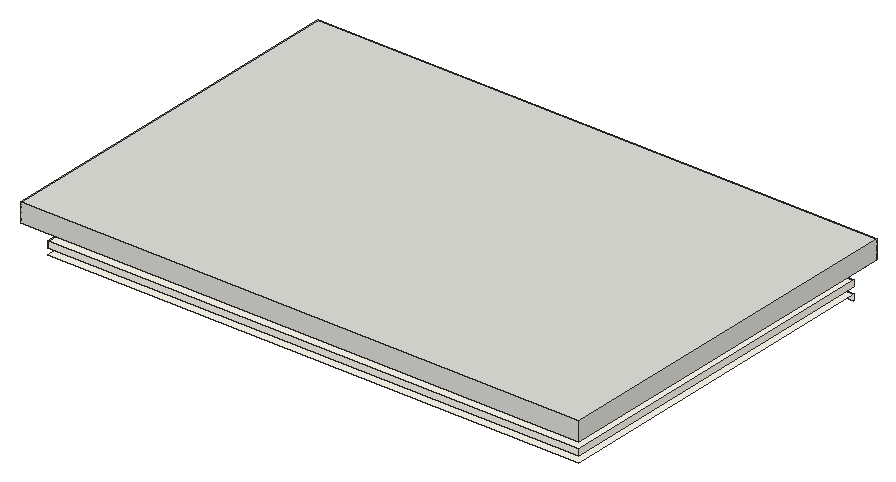
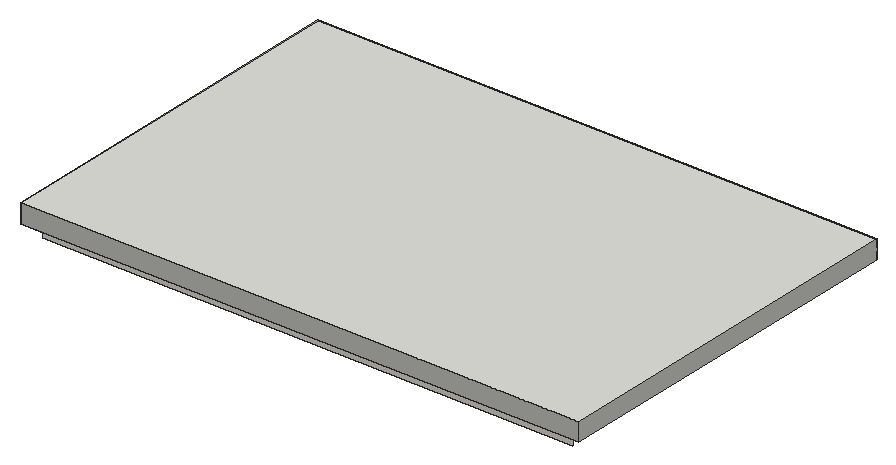
# SketchUp Ruby script. Lengths in inches.
U = 1.inch
M = Sketchup.active_model
def pt(a) = Geom::Point3d.new(a.map { |v| v * U })
def face(e, loops, mat)
  f = e.add_face(loops[0].map { |a| pt(a) })
  loops[1..].each { |l| e.add_face(l.map { |a| pt(a) }).erase! }
  f.material = f.back_material = mat if mat
  f
end
# faces: each face lists its corners as indices into pts; further lists are holes
def faces(e, pts, list, mat = nil) = list.each { |f| face(e, (f[0].is_a?(Array) ? f : [f]).map { |l| l.map { |i| pts[i] } }, mat) }
# xy, xz, yz: faces in a plane at the given z, y or x. An outline is a flat list of corners, or four numbers for a rectangle; further outlines are holes
def ring(l) = l.size == 4 ? [[l[0], l[1]], [l[2], l[1]], [l[2], l[3]], [l[0], l[3]]] : l.each_slice(2).to_a
def flat(e, list, mat, &to3) = list.each { |f| face(e, (f[0].is_a?(Array) ? f : [f]).map { |l| ring(l).map { |u, v| to3.(u, v) } }, mat) }
def xy(e, z, list, mat = nil) = flat(e, list, mat) { |x, y| [x, y, z] }
def xz(e, y, list, mat = nil) = flat(e, list, mat) { |x, z| [x, y, z] }
def yz(e, x, list, mat = nil) = flat(e, list, mat) { |y, z| [x, y, z] }
def lines(e, pts, list) = list.each { |a, b| e.add_line(pt(pts[a]), pt(pts[b])) }
# prism: a flat outline (further loops are holes) pulled along v
def prism(e, loops, v, mat = nil)
  f = face(e, loops, mat); d = Geom::Vector3d.new(v.map { |x| x * U })
  f.pushpull(f.normal.samedirection?(d) ? d.length : -d.length)
end
def box(e, o, s, mat = nil) = prism(e, [[o, [o[0] + s[0], o[1], o[2]], [o[0] + s[0], o[1] + s[1], o[2]], [o[0], o[1] + s[1], o[2]]]], [0, 0, s[2]], mat)
def at(x, y, z, deg = 0) = Geom::Transformation.translation(pt([x, y, z])) * Geom::Transformation.rotation(ORIGIN, Z_AXIS, deg.degrees)
def axes(o, x, y, z) = Geom::Transformation.new([*x, 0, *y, 0, *z, 0, *pt(o).to_a, 1])
def part(name) = M.definitions.add(name)
# library, detail: a bought-in or finely detailed component or shape, given as its bounding box
def library(name, o, s) = part(name).tap { |d| box(d.entities, o, s) }
def detail(e, o, s) = box(e.add_group.entities, o, s)
def put(e, d, t, mat = nil) = e.add_instance(d, t).tap { |i| i.material = mat if mat }
def group(e, t, mat = nil) = e.add_group.tap { |g| g.transformation = t; g.material = mat if mat }.entities
root = M.entities
M.materials.add("[0052_FloralWhite]").color = [255, 250, 240]
M.materials.add("[Color D02]").color = [214, 192, 128]
M.materials.add("[Color E02]").color = [255, 255, 153]
M.materials.add("[Metal Aluminum Anodized]").color = [202, 209, 219]
xy(root,118.125,[[[49.94,94.53,49.875,94.55,49.81,94.5625,49.74,94.58,49.67,94.61,49.61,94.64,49.55,94.68,49.49,94.71,49.4375,94.76,49.39,94.8,49.34,94.85,49.29,94.91,49.25,94.96,49.21,95.02,49.18,95.08,49.15,95.15,49.13,95.21,49.09,95.35,49.08,95.42,49.08,95.63,49.09,95.7,49.11,95.76,49.15,95.9,49.21,96.02,49.29,96.14,49.33,96.19,49.43,96.29,49.61,96.41,49.67,96.4375,49.73,96.46,49.8,96.49,49.87,96.5,49.9375,96.51,50.01,96.52,50.22,96.52,50.28,96.5,50.35,96.49,50.42,96.47,50.48,96.44,50.55,96.41,50.61,96.375,50.66,96.34,50.72,96.29,50.77,96.25,50.82,96.2,50.87,96.14,50.91,96.09,50.94,96.03,50.98,95.97,51.01,95.9,51.03,95.84,51.05,95.77,51.0625,95.7,51.07,95.63,51.08,95.5625,51.08,95.49,51.07,95.42,51.0625,95.35,51.05,95.29,51.01,95.15,50.95,95.03,50.87,94.91,50.82,94.86,50.78,94.81,50.72,94.76,50.67,94.72,50.55,94.64,50.49,94.61,50.42,94.59,50.36,94.5625,50.29,94.55,50.15,94.53],[50.02,94.7,50.14,94.7,50.2,94.71,50.25,94.72,50.31,94.73,50.36,94.75,50.42,94.77,50.52,94.83,50.56,94.86,50.61,94.9,50.65,94.93,50.69,94.98,50.73,95.02,50.76,95.07,50.79,95.11,50.82,95.17,50.86,95.27,50.88,95.33,50.89,95.38,50.9,95.44,50.9,95.61,50.88,95.73,50.86,95.78,50.84,95.84,50.82,95.89,50.79,95.9375,50.76,95.99,50.73,96.03,50.69,96.08,50.61,96.16,50.5625,96.19,50.51,96.22,50.41,96.28,50.36,96.3,50.3,96.32,50.25,96.33,50.13,96.35,50.02,96.35,49.96,96.34,49.91,96.33,49.85,96.32,49.8,96.3,49.74,96.28,49.59,96.19,49.55,96.15,49.5,96.12,49.47,96.07,49.43,96.03,49.39,95.98,49.36,95.94,49.34,95.88,49.3125,95.83,49.29,95.78,49.28,95.72,49.27,95.67,49.26,95.61,49.26,95.4375,49.27,95.38,49.28,95.32,49.3,95.27,49.32,95.21,49.34,95.16,49.37,95.11,49.4,95.0625,49.43,95.02,49.47,94.97,49.55,94.89,49.6,94.86,49.64,94.83,49.69,94.8,49.75,94.77,49.85,94.73,49.97,94.71]]],"[Metal Aluminum Anodized]")
xy(root,118.1875,[[50.02,94.7,49.97,94.71,49.85,94.73,49.75,94.77,49.69,94.8,49.64,94.83,49.6,94.86,49.55,94.89,49.47,94.97,49.43,95.02,49.4,95.0625,49.37,95.11,49.34,95.16,49.32,95.21,49.3,95.27,49.28,95.32,49.27,95.38,49.26,95.4375,49.26,95.61,49.27,95.67,49.28,95.72,49.29,95.78,49.3125,95.83,49.34,95.88,49.36,95.94,49.39,95.98,49.43,96.03,49.47,96.07,49.5,96.12,49.55,96.15,49.59,96.19,49.74,96.28,49.8,96.3,49.85,96.32,49.91,96.33,49.96,96.34,50.02,96.35,50.13,96.35,50.25,96.33,50.3,96.32,50.36,96.3,50.41,96.28,50.51,96.22,50.5625,96.19,50.61,96.16,50.69,96.08,50.73,96.03,50.76,95.99,50.79,95.9375,50.82,95.89,50.84,95.84,50.86,95.78,50.88,95.73,50.9,95.61,50.9,95.44,50.89,95.38,50.88,95.33,50.86,95.27,50.82,95.17,50.79,95.11,50.76,95.07,50.73,95.02,50.69,94.98,50.65,94.93,50.61,94.9,50.56,94.86,50.52,94.83,50.42,94.77,50.36,94.75,50.31,94.73,50.25,94.72,50.2,94.71,50.14,94.7]],"[Color D02]")
xy(root,118.3,[[[24.3,77.95,24.23,77.96,24.16,77.96,24.09,77.98,24.02,77.99,23.96,78.01,23.89,78.04,23.83,78.07,23.77,78.11,23.71,78.14,23.66,78.1875,23.61,78.23,23.56,78.28,23.51,78.34,23.47,78.39,23.43,78.45,23.4,78.52,23.37,78.58,23.35,78.64,23.33,78.71,23.3,78.92,23.3,78.99,23.33,79.2,23.35,79.26,23.37,79.33,23.43,79.45,23.51,79.57,23.66,79.72,23.71,79.76,23.83,79.84,23.89,79.87,23.96,79.89,24.02,79.92,24.23,79.95,24.37,79.95,24.4375,79.94,24.51,79.93,24.58,79.92,24.64,79.89,24.71,79.87,24.77,79.84,24.89,79.76,24.94,79.72,25.09,79.57,25.17,79.45,25.23,79.33,25.25,79.26,25.27,79.2,25.3,78.99,25.3,78.92,25.27,78.71,25.25,78.64,25.23,78.58,25.2,78.52,25.17,78.45,25.13,78.39,25.09,78.34,25.04,78.28,24.99,78.23,24.94,78.1875,24.89,78.14,24.83,78.11,24.77,78.07,24.71,78.04,24.64,78.01,24.58,77.99,24.51,77.98,24.4375,77.96,24.37,77.96],[24.23,78.02,24.37,78.02,24.49,78.04,24.56,78.06,24.68,78.1,24.74,78.13,24.79,78.16,24.85,78.2,24.95,78.28,24.99,78.33,25.04,78.38,25.07,78.43,25.11,78.49,25.14,78.54,25.16,78.6,25.1875,78.67,25.21,78.73,25.22,78.79,25.23,78.86,25.23,79.05,25.22,79.12,25.21,79.18,25.1875,79.24,25.16,79.3,25.14,79.36,25.11,79.42,25.07,79.48,25.04,79.53,24.99,79.58,24.95,79.625,24.9,79.67,24.85,79.71,24.79,79.74,24.74,79.78,24.68,79.81,24.56,79.85,24.49,79.87,24.43,79.88,24.37,79.88,24.3,79.89,24.23,79.88,24.17,79.88,24.11,79.87,24.04,79.85,23.92,79.81,23.86,79.78,23.81,79.74,23.75,79.71,23.7,79.67,23.65,79.625,23.61,79.58,23.56,79.53,23.53,79.48,23.49,79.42,23.46,79.36,23.44,79.3,23.41,79.24,23.39,79.18,23.38,79.12,23.37,79.05,23.37,78.86,23.38,78.79,23.39,78.73,23.41,78.67,23.44,78.6,23.46,78.54,23.49,78.49,23.53,78.43,23.56,78.38,23.61,78.33,23.65,78.28,23.75,78.2,23.81,78.16,23.86,78.13,23.92,78.1,24.04,78.06,24.11,78.04]]],"[Metal Aluminum Anodized]")
xy(root,118.375,[[24.23,78.02,24.11,78.04,24.04,78.06,23.92,78.1,23.86,78.13,23.81,78.16,23.75,78.2,23.65,78.28,23.61,78.33,23.56,78.38,23.53,78.43,23.49,78.49,23.46,78.54,23.44,78.6,23.41,78.67,23.39,78.73,23.38,78.79,23.37,78.86,23.37,79.05,23.38,79.12,23.39,79.18,23.41,79.24,23.44,79.3,23.46,79.36,23.49,79.42,23.53,79.48,23.56,79.53,23.61,79.58,23.65,79.625,23.7,79.67,23.75,79.71,23.81,79.74,23.86,79.78,23.92,79.81,24.04,79.85,24.11,79.87,24.17,79.88,24.23,79.88,24.3,79.89,24.37,79.88,24.43,79.88,24.49,79.87,24.56,79.85,24.68,79.81,24.74,79.78,24.79,79.74,24.85,79.71,24.9,79.67,24.95,79.625,24.99,79.58,25.04,79.53,25.07,79.48,25.11,79.42,25.14,79.36,25.16,79.3,25.1875,79.24,25.21,79.18,25.22,79.12,25.23,79.05,25.23,78.86,25.22,78.79,25.21,78.73,25.1875,78.67,25.16,78.6,25.14,78.54,25.11,78.49,25.07,78.43,25.04,78.38,24.99,78.33,24.95,78.28,24.85,78.2,24.79,78.16,24.74,78.13,24.68,78.1,24.56,78.06,24.49,78.04,24.37,78.02]],"[Color E02]")
xy(root,120,[[[9,0,180,111],[39.6,30.6,149.4,80.4]]],"[0052_FloralWhite]")
xz(root,78.02,[[24.23,118.3,24.3,118.375],[24.3,118.3,24.37,118.375]],"[0052_FloralWhite]")
xz(root,79.88,[[24.17,118.3,24.23,118.375],[24.37,118.3,24.43,118.375]],"[0052_FloralWhite]")
xz(root,79.95,[[24.23,118,24.3,118.3],[24.3,118,24.37,118.3]],"[Metal Aluminum Anodized]")
xz(root,94.7,[[50.02,118.125,50.08,118.1875],[50.08,118.125,50.14,118.1875]],"[Metal Aluminum Anodized]")
xz(root,96.35,[[50.02,118.125,50.08,118.1875],[50.08,118.125,50.13,118.1875]],"[Metal Aluminum Anodized]")
xz(root,111,[[9,118,180,120]],"[0052_FloralWhite]")
yz(root,23.37,[[78.86,118.3,78.92,118.375],[78.92,118.3,78.99,118.375],[78.99,118.3,79.05,118.375]],"[0052_FloralWhite]")
yz(root,25.23,[[78.86,118.3,78.92,118.375],[78.92,118.3,78.99,118.375],[78.99,118.3,79.05,118.375]],"[0052_FloralWhite]")
yz(root,49.26,[[95.4375,118.125,95.49,118.1875],[95.49,118.125,95.55,118.1875],[95.55,118.125,95.61,118.1875]],"[Metal Aluminum Anodized]")
yz(root,50.9,[[95.44,118.125,95.5,118.1875],[95.5,118.125,95.56,118.1875],[95.56,118.125,95.61,118.1875]],"[Metal Aluminum Anodized]")
p = [[23.66,79.72,118],[23.71,79.76,118],[23.71,79.76,118.3],[23.66,79.72,118.3],[24.89,79.76,118],[24.94,79.72,118],
  [24.94,79.72,118.3],[24.89,79.76,118.3],[23.77,79.8,118],[23.77,79.8,118.3],[23.83,79.84,118],[23.83,79.84,118.3],
  [23.89,79.87,118],[23.89,79.87,118.3],[24.71,79.87,118],[24.77,79.84,118],[24.77,79.84,118.3],[24.71,79.87,118.3],
  [24.83,79.8,118],[24.83,79.8,118.3],[23.96,79.89,118],[23.96,79.89,118.3],[24.02,79.92,118],[24.02,79.92,118.3],
  [24.09,79.93,118],[24.09,79.93,118.3],[24.16,79.94,118],[24.16,79.94,118.3],[24.23,79.95,118],[24.23,79.95,118.3],
  [24.37,79.95,118],[24.4375,79.94,118],[24.4375,79.94,118.3],[24.37,79.95,118.3],[24.51,79.93,118],[24.51,79.93,118.3],
  [24.58,79.92,118],[24.58,79.92,118.3],[24.64,79.89,118],[24.64,79.89,118.3],[49.8,94.75,118.1875],[49.8,94.75,118.125],
  [49.75,94.77,118.125],[49.75,94.77,118.1875],[49.85,94.73,118.1875],[49.85,94.73,118.125],[49.97,94.71,118.1875],[49.97,94.71,118.125],
  [49.91,94.72,118.125],[49.91,94.72,118.1875],[50.02,94.7,118.1875],[50.02,94.7,118.125],[50.2,94.71,118.1875],[50.2,94.71,118.125],
  [50.14,94.7,118.125],[50.14,94.7,118.1875],[50.25,94.72,118.1875],[50.25,94.72,118.125],[50.36,94.75,118.1875],[50.36,94.75,118.125],
  [50.31,94.73,118.125],[50.31,94.73,118.1875],[49.69,94.8,118.1875],[49.69,94.8,118.125],[49.64,94.83,118.125],[49.64,94.83,118.1875],
  [49.6,94.86,118.125],[49.6,94.86,118.1875],[50.47,94.8,118.1875],[50.47,94.8,118.125],[50.42,94.77,118.125],[50.42,94.77,118.1875],
  [50.56,94.86,118.1875],[50.56,94.86,118.125],[50.52,94.83,118.125],[50.52,94.83,118.1875],[49.55,94.89,118.1875],[49.55,94.89,118.125],
  [49.51,94.93,118.125],[49.51,94.93,118.1875],[49.47,94.97,118.125],[49.47,94.97,118.1875],[50.65,94.93,118.1875],[50.65,94.93,118.125],
  [50.61,94.9,118.125],[50.61,94.9,118.1875],[50.69,94.98,118.1875],[50.69,94.98,118.125],[49.43,95.02,118.125],[49.43,95.02,118.1875],
  [49.4,95.0625,118.125],[49.4,95.0625,118.1875],[50.76,95.07,118.1875],[50.76,95.07,118.125],[50.73,95.02,118.125],[50.73,95.02,118.1875],
  [49.37,95.11,118.1875],[49.37,95.11,118.125],[49.34,95.16,118.125],[49.34,95.16,118.1875],[50.82,95.17,118.1875],[50.82,95.17,118.125],
  [50.79,95.11,118.125],[50.79,95.11,118.1875],[49.32,95.21,118.125],[49.32,95.21,118.1875],[49.3,95.27,118.125],[49.3,95.27,118.1875],
  [50.86,95.27,118.1875],[50.86,95.27,118.125],[50.84,95.22,118.125],[50.84,95.22,118.1875],[49.28,95.32,118.125],[49.28,95.32,118.1875],
  [49.27,95.38,118.125],[49.27,95.38,118.1875],[50.89,95.38,118.1875],[50.89,95.38,118.125],[50.88,95.33,118.125],[50.88,95.33,118.1875],
  [49.26,95.4375,118.125],[49.26,95.4375,118.1875],[50.9,95.44,118.1875],[50.9,95.44,118.125],[49.26,95.61,118.1875],[49.26,95.61,118.125],
  [49.27,95.67,118.125],[49.27,95.67,118.1875],[50.89,95.67,118.1875],[50.89,95.67,118.125],[50.9,95.61,118.125],[50.9,95.61,118.1875],
  [49.28,95.72,118.125],[49.28,95.72,118.1875],[49.29,95.78,118.125],[49.29,95.78,118.1875],[50.86,95.78,118.1875],[50.86,95.78,118.125],
  [50.88,95.73,118.125],[50.88,95.73,118.1875],[49.3125,95.83,118.125],[49.3125,95.83,118.1875],[49.34,95.88,118.125],[49.34,95.88,118.1875],
  [50.82,95.89,118.1875],[50.82,95.89,118.125],[50.84,95.84,118.125],[50.84,95.84,118.1875],[49.36,95.94,118.125],[49.36,95.94,118.1875],
  [49.39,95.98,118.125],[49.39,95.98,118.1875],[50.76,95.99,118.1875],[50.76,95.99,118.125],[50.79,95.9375,118.125],[50.79,95.9375,118.1875],
  [49.43,96.03,118.125],[49.43,96.03,118.1875],[49.47,96.07,118.125],[49.47,96.07,118.1875],[50.69,96.08,118.1875],[50.69,96.08,118.125],
  [50.73,96.03,118.125],[50.73,96.03,118.1875],[49.5,96.12,118.125],[49.5,96.12,118.1875],[49.55,96.15,118.125],[49.55,96.15,118.1875],
  [50.61,96.16,118.1875],[50.61,96.16,118.125],[50.65,96.12,118.125],[50.65,96.12,118.1875],[49.59,96.19,118.125],[49.59,96.19,118.1875],
  [49.64,96.22,118.125],[49.64,96.22,118.1875],[49.69,96.25,118.125],[49.69,96.25,118.1875],[50.46,96.25,118.1875],[50.46,96.25,118.125],
  [50.51,96.22,118.125],[50.51,96.22,118.1875],[50.5625,96.19,118.125],[50.5625,96.19,118.1875],[49.74,96.28,118.125],[49.74,96.28,118.1875],
  [49.8,96.3,118.125],[49.8,96.3,118.1875],[49.85,96.32,118.125],[49.85,96.32,118.1875],[49.91,96.33,118.125],[49.91,96.33,118.1875],
  [49.96,96.34,118.125],[49.96,96.34,118.1875],[50.02,96.35,118.125],[50.02,96.35,118.1875],[50.13,96.35,118.1875],[50.13,96.35,118.125],
  [50.19,96.34,118.125],[50.19,96.34,118.1875],[50.25,96.33,118.125],[50.25,96.33,118.1875],[50.3,96.32,118.125],[50.3,96.32,118.1875],
  [50.36,96.3,118.125],[50.36,96.3,118.1875],[50.41,96.28,118.125],[50.41,96.28,118.1875],[24.11,78.04,118.375],[24.11,78.04,118.3],
  [24.04,78.06,118.3],[24.04,78.06,118.375],[24.17,78.03,118.375],[24.17,78.03,118.3],[24.23,78.02,118.375],[24.23,78.02,118.3],
  [24.49,78.04,118.375],[24.49,78.04,118.3],[24.43,78.03,118.3],[24.43,78.03,118.375],[24.37,78.02,118.3],[24.37,78.02,118.375],
  [24.56,78.06,118.375],[24.56,78.06,118.3],[23.86,78.13,118.375],[23.86,78.13,118.3],[23.81,78.16,118.3],[23.81,78.16,118.375],
  [23.98,78.08,118.375],[23.98,78.08,118.3],[23.92,78.1,118.3],[23.92,78.1,118.375],[24.68,78.1,118.375],[24.68,78.1,118.3],
  [24.62,78.08,118.3],[24.62,78.08,118.375],[24.79,78.16,118.375],[24.79,78.16,118.3],[24.74,78.13,118.3],[24.74,78.13,118.375],
  [23.75,78.2,118.375],[23.75,78.2,118.3],[23.7,78.24,118.3],[23.7,78.24,118.375],[23.65,78.28,118.3],[23.65,78.28,118.375],
  [24.9,78.24,118.375],[24.9,78.24,118.3],[24.85,78.2,118.3],[24.85,78.2,118.375],[24.95,78.28,118.375],[24.95,78.28,118.3],
  [23.61,78.33,118.3],[23.61,78.33,118.375],[23.56,78.38,118.3],[23.56,78.38,118.375],[24.99,78.33,118.375],[24.99,78.33,118.3],
  [25.04,78.38,118.375],[25.04,78.38,118.3],[23.53,78.43,118.3],[23.53,78.43,118.375],[23.49,78.49,118.3],[23.49,78.49,118.375],
  [25.07,78.43,118.375],[25.07,78.43,118.3],[25.11,78.49,118.375],[25.11,78.49,118.3],[23.46,78.54,118.375],[23.46,78.54,118.3],
  [23.44,78.6,118.3],[23.44,78.6,118.375],[25.16,78.6,118.375],[25.16,78.6,118.3],[25.14,78.54,118.3],[25.14,78.54,118.375],
  [23.41,78.67,118.3],[23.41,78.67,118.375],[25.1875,78.67,118.375],[25.1875,78.67,118.3],[23.39,78.73,118.3],[23.39,78.73,118.375],
  [23.38,78.79,118.3],[23.38,78.79,118.375],[25.21,78.73,118.375],[25.21,78.73,118.3],[25.22,78.79,118.375],[25.22,78.79,118.3],
  [23.37,78.86,118.3],[23.37,78.86,118.375],[25.23,78.86,118.375],[25.23,78.86,118.3],[23.37,79.05,118.375],[23.37,79.05,118.3],
  [23.38,79.12,118.3],[23.38,79.12,118.375],[23.39,79.18,118.3],[23.39,79.18,118.375],[25.21,79.18,118.375],[25.21,79.18,118.3],
  [25.22,79.12,118.3],[25.22,79.12,118.375],[25.23,79.05,118.3],[25.23,79.05,118.375],[23.41,79.24,118.3],[23.41,79.24,118.375],
  [23.44,79.3,118.3],[23.44,79.3,118.375],[25.1875,79.24,118.375],[25.1875,79.24,118.3],[25.16,79.3,118.375],[25.16,79.3,118.3],
  [23.46,79.36,118.3],[23.46,79.36,118.375],[25.14,79.36,118.375],[25.14,79.36,118.3],[23.49,79.42,118.3],[23.49,79.42,118.375],
  [23.53,79.48,118.3],[23.53,79.48,118.375],[25.07,79.48,118.375],[25.07,79.48,118.3],[25.11,79.42,118.3],[25.11,79.42,118.375],
  [23.56,79.53,118.3],[23.56,79.53,118.375],[23.61,79.58,118.3],[23.61,79.58,118.375],[24.99,79.58,118.375],[24.99,79.58,118.3],
  [25.04,79.53,118.3],[25.04,79.53,118.375],[23.65,79.625,118.3],[23.65,79.625,118.375],[23.7,79.67,118.3],[23.7,79.67,118.375],
  [24.9,79.67,118.375],[24.9,79.67,118.3],[24.95,79.625,118.3],[24.95,79.625,118.375],[23.75,79.71,118.3],[23.75,79.71,118.375],
  [23.81,79.74,118.3],[23.81,79.74,118.375],[23.86,79.78,118.3],[23.86,79.78,118.375],[24.74,79.78,118.375],[24.74,79.78,118.3],
  [24.79,79.74,118.3],[24.79,79.74,118.375],[24.85,79.71,118.3],[24.85,79.71,118.375],[23.92,79.81,118.3],[23.92,79.81,118.375],
  [23.98,79.83,118.3],[23.98,79.83,118.375],[24.04,79.85,118.3],[24.04,79.85,118.375],[24.56,79.85,118.375],[24.56,79.85,118.3],
  [24.62,79.83,118.3],[24.62,79.83,118.375],[24.68,79.81,118.3],[24.68,79.81,118.375],[24.11,79.87,118.3],[24.11,79.87,118.375],
  [24.17,79.88,118.3],[24.17,79.88,118.375],[24.23,79.88,118.375],[24.23,79.88,118.3],[24.3,79.89,118.3],[24.3,79.89,118.375],
  [24.37,79.88,118.3],[24.37,79.88,118.375],[24.43,79.88,118.375],[24.43,79.88,118.3],[24.49,79.87,118.3],[24.49,79.87,118.375]]
faces(root,p,[[0,1,2,3],[4,5,6,7],[1,8,9,2],[8,10,11,9],[10,12,13,11],[14,15,16,17],[15,18,19,16],[18,4,7,19],
  [12,20,21,13],[20,22,23,21],[22,24,25,23],[24,26,27,25],[26,28,29,27],[30,31,32,33],[31,34,35,32],[34,36,37,35],
  [36,38,39,37],[38,14,17,39],[40,41,42,43],[44,45,41,40],[46,47,48,49],[49,48,45,44],[50,51,47,46],[52,53,54,55],
  [56,57,53,52],[58,59,60,61],[61,60,57,56],[62,63,64,65],[65,64,66,67],[43,42,63,62],[68,69,70,71],[71,70,59,58],
  [72,73,74,75],[75,74,69,68],[76,77,78,79],[79,78,80,81],[67,66,77,76],[82,83,84,85],[85,84,73,72],[86,87,83,82],
  [81,80,88,89],[89,88,90,91],[92,93,94,95],[95,94,87,86],[96,97,98,99],[91,90,97,96],[100,101,102,103],[103,102,93,92],
  [99,98,104,105],[105,104,106,107],[108,109,110,111],[111,110,101,100],[107,106,112,113],[113,112,114,115],[116,117,118,119],[119,118,109,108],
  [115,114,120,121],[122,123,117,116],[124,125,126,127],[128,129,130,131],[127,126,132,133],[133,132,134,135],[136,137,138,139],[139,138,129,128],
  [135,134,140,141],[141,140,142,143],[144,145,146,147],[147,146,137,136],[143,142,148,149],[149,148,150,151],[152,153,154,155],[155,154,145,144],
  [151,150,156,157],[157,156,158,159],[160,161,162,163],[163,162,153,152],[159,158,164,165],[165,164,166,167],[168,169,170,171],[171,170,161,160],
  [167,166,172,173],[173,172,174,175],[175,174,176,177],[178,179,180,181],[181,180,182,183],[183,182,169,168],[177,176,184,185],[185,184,186,187],
  [187,186,188,189],[189,188,190,191],[191,190,192,193],[193,192,194,195],[196,197,198,199],[199,198,200,201],[201,200,202,203],[203,202,204,205],
  [205,204,206,207],[207,206,179,178]],"[Metal Aluminum Anodized]")
faces(root,p,[[208,209,210,211],[212,213,209,208],[214,215,213,212],[216,217,218,219],[219,218,220,221],[222,223,217,216],[224,225,226,227],[228,229,230,231],
  [231,230,225,224],[211,210,229,228],[232,233,234,235],[235,234,223,222],[236,237,238,239],[239,238,233,232],[240,241,242,243],[243,242,244,245],
  [227,226,241,240],[246,247,248,249],[249,248,237,236],[250,251,247,246],[245,244,252,253],[253,252,254,255],[256,257,251,250],[258,259,257,256],
  [255,254,260,261],[261,260,262,263],[264,265,259,258],[266,267,265,264],[268,269,270,271],[263,262,269,268],[272,273,274,275],[275,274,267,266],
  [271,270,276,277],[278,279,273,272],[277,276,280,281],[281,280,282,283],[284,285,279,278],[286,287,285,284],[283,282,288,289],[290,291,287,286],
  [292,293,294,295],[295,294,296,297],[298,299,300,301],[301,300,302,303],[297,296,304,305],[305,304,306,307],[308,309,299,298],[310,311,309,308],
  [307,306,312,313],[314,315,311,310],[313,312,316,317],[317,316,318,319],[320,321,322,323],[323,322,315,314],[319,318,324,325],[325,324,326,327],
  [328,329,330,331],[331,330,321,320],[327,326,332,333],[333,332,334,335],[336,337,338,339],[339,338,329,328],[335,334,340,341],[341,340,342,343],
  [343,342,344,345],[346,347,348,349],[349,348,350,351],[351,350,337,336],[345,344,352,353],[353,352,354,355],[355,354,356,357],[358,359,360,361],
  [361,360,362,363],[363,362,347,346],[357,356,364,365],[365,364,366,367],[368,369,370,371],[371,370,372,373],[374,375,376,377],[377,376,359,358]],"[0052_FloralWhite]")
g1 = group(root,at(9,0,122),"[0052_FloralWhite]")
box(g1,[0,0,0],[171,111,2])
g2 = group(root,at(0,0,126))
box(g2,[0,0,0],[180,120,6])
